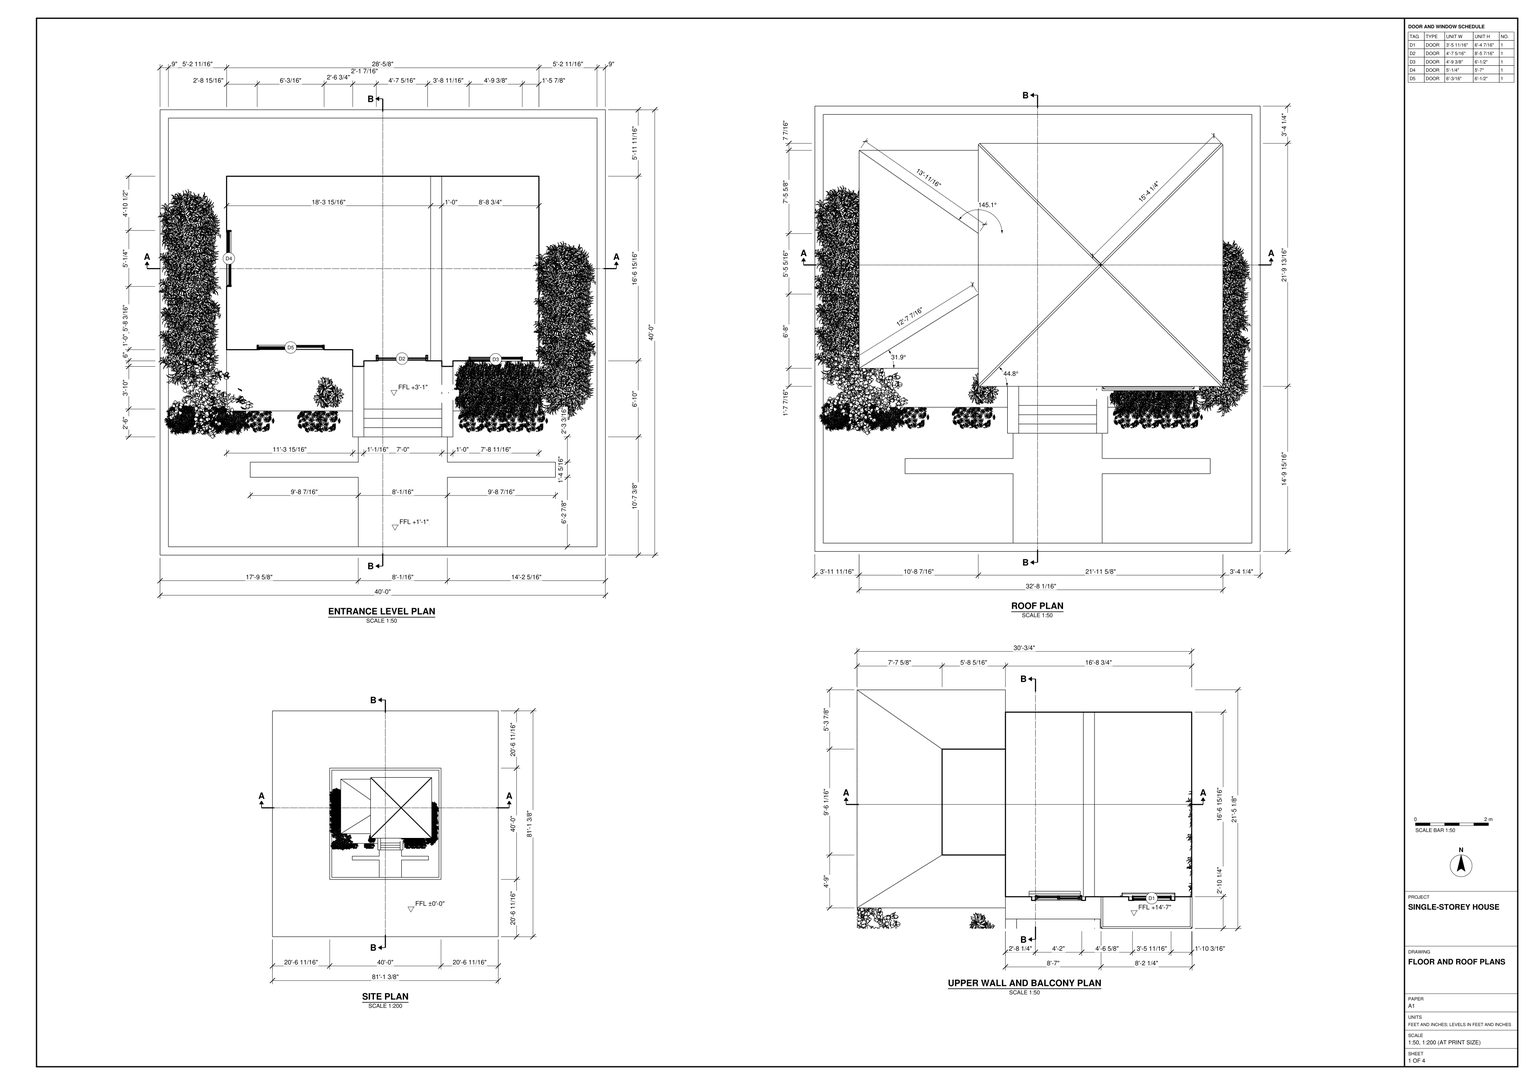
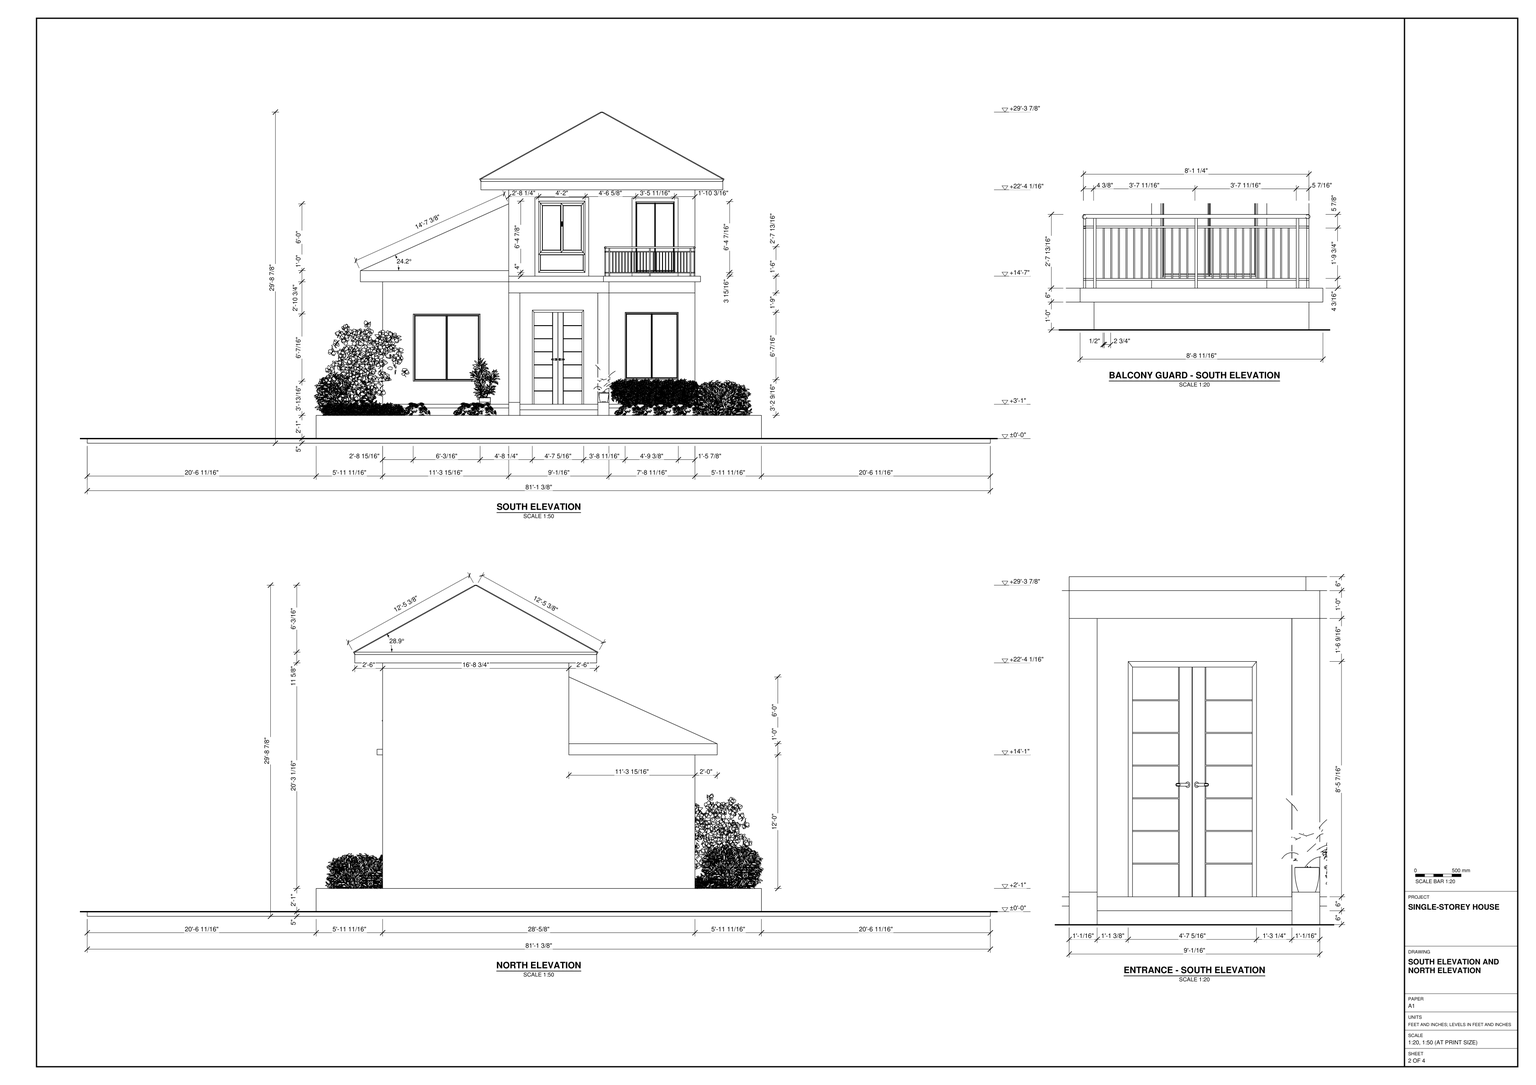
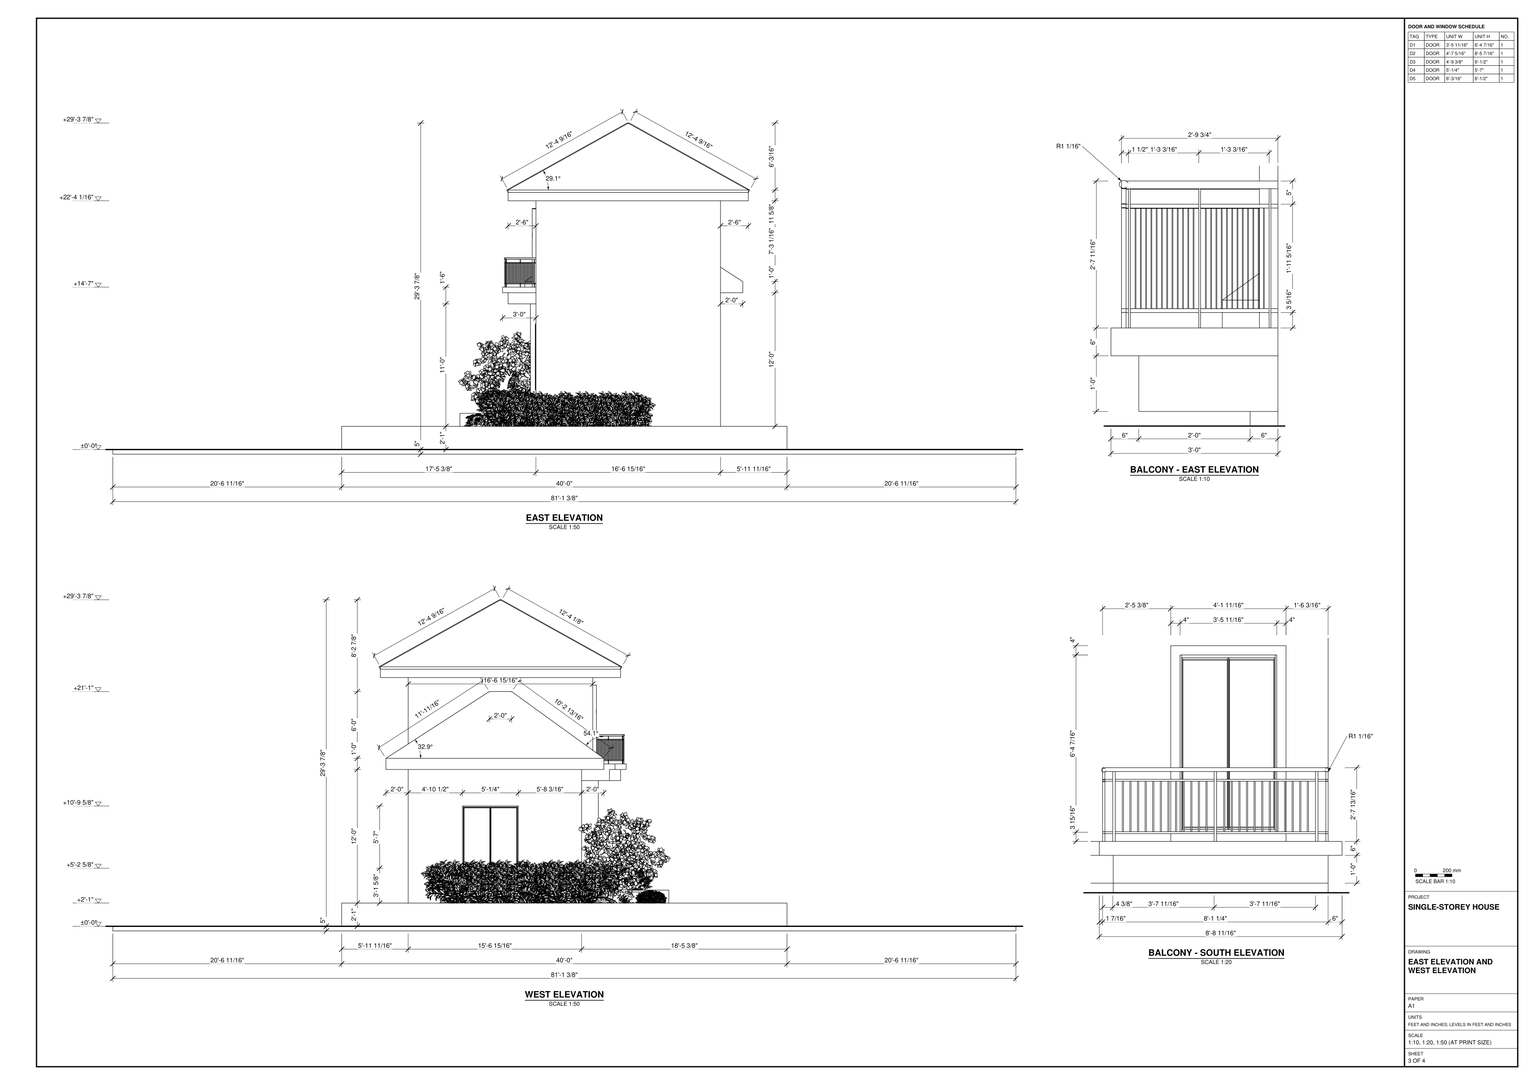
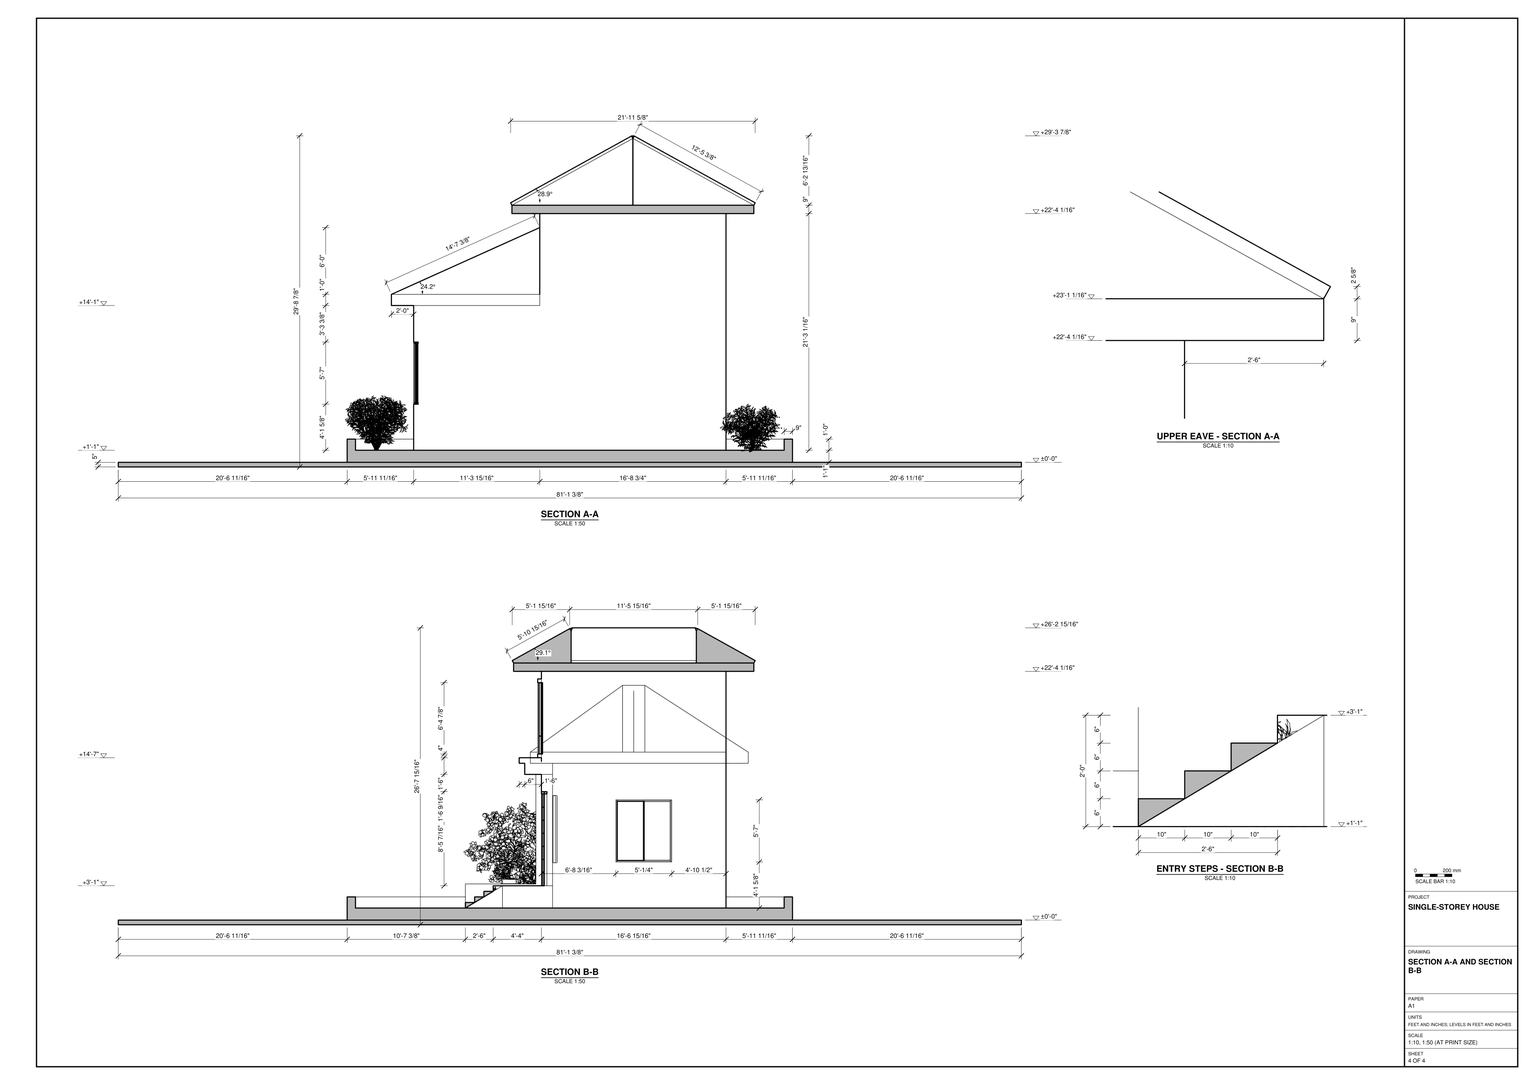
Build the house and its site in SketchUp from task_files/diagram_01.pdf. Work in feet and inches. Use the site datum of ±0'-0". The complete model, including the base slab, must measure 81'-1 3/8" along both plan axes and 29'-8 7/8" from the underside of the base to the roof peak.

Centre the raised square plot on the larger site slab. Run the entrance path from the south edge of the plot to the steps and landing at the double entrance door. Follow the entrance plan for the wall positions and thicknesses, the offsets in the south facade and the widths of the openings. Fit the glazed units on either side of the entrance and in the west wall. Model the upper south window and the door onto the projecting balcony, including its slab, front guard and side returns.

Form the taller east roof with hips meeting at a single peak. Fit the lower west roof against the taller wall, matching the roof plan and the eave profiles in elevation. Place the planting in the beds shown around the house. Plants, decor and loose items may be suitable library components. Keep walls, slabs, roofs and individual joinery or furniture pieces in separate groups or components, and use components for repeated parts. Save one SketchUp model as output_files/single_storey_house_with_hipped_roofs_and_a_balcony.skp.

# SketchUp Ruby script. Lengths in inches.
U = 1.inch
M = Sketchup.active_model
def pt(a) = Geom::Point3d.new(a.map { |v| v * U })
def face(e, loops, mat)
  f = e.add_face(loops[0].map { |a| pt(a) })
  loops[1..].each { |l| e.add_face(l.map { |a| pt(a) }).erase! }
  f.material = f.back_material = mat if mat
  f
end
# faces: each face lists its corners as indices into pts; further lists are holes
def faces(e, pts, list, mat = nil) = list.each { |f| face(e, (f[0].is_a?(Array) ? f : [f]).map { |l| l.map { |i| pts[i] } }, mat) }
# xy, xz, yz: faces in a plane at the given z, y or x. An outline is a flat list of corners, or four numbers for a rectangle; further outlines are holes
def ring(l) = l.size == 4 ? [[l[0], l[1]], [l[2], l[1]], [l[2], l[3]], [l[0], l[3]]] : l.each_slice(2).to_a
def flat(e, list, mat, &to3) = list.each { |f| face(e, (f[0].is_a?(Array) ? f : [f]).map { |l| ring(l).map { |u, v| to3.(u, v) } }, mat) }
def xy(e, z, list, mat = nil) = flat(e, list, mat) { |x, y| [x, y, z] }
def xz(e, y, list, mat = nil) = flat(e, list, mat) { |x, z| [x, y, z] }
def yz(e, x, list, mat = nil) = flat(e, list, mat) { |y, z| [x, y, z] }
def lines(e, pts, list) = list.each { |a, b| e.add_line(pt(pts[a]), pt(pts[b])) }
# prism: a flat outline (further loops are holes) pulled along v
def prism(e, loops, v, mat = nil)
  f = face(e, loops, mat); d = Geom::Vector3d.new(v.map { |x| x * U })
  f.pushpull(f.normal.samedirection?(d) ? d.length : -d.length)
end
def box(e, o, s, mat = nil) = prism(e, [[o, [o[0] + s[0], o[1], o[2]], [o[0] + s[0], o[1] + s[1], o[2]], [o[0], o[1] + s[1], o[2]]]], [0, 0, s[2]], mat)
def at(x, y, z, deg = 0) = Geom::Transformation.translation(pt([x, y, z])) * Geom::Transformation.rotation(ORIGIN, Z_AXIS, deg.degrees)
def axes(o, x, y, z) = Geom::Transformation.new([*x, 0, *y, 0, *z, 0, *pt(o).to_a, 1])
def part(name) = M.definitions.add(name)
# library, detail: a bought-in or finely detailed component or shape, given as its bounding box
def library(name, o, s) = part(name).tap { |d| box(d.entities, o, s) }
def detail(e, o, s) = box(e.add_group.entities, o, s)
def put(e, d, t, mat = nil) = e.add_instance(d, t).tap { |i| i.material = mat if mat }
def group(e, t, mat = nil) = e.add_group.tap { |g| g.transformation = t; g.material = mat if mat }.entities
root = M.entities
M.materials.add("Glass_Tinted_Gray").color = [0, 0, 0]
M.materials["Glass_Tinted_Gray"].alpha = 0.125
M.materials.add("[0045_Goldenrod]").color = [218, 165, 32]
M.materials.add("[0053_Ivory]").color = [255, 255, 240]
M.materials.add("[0135_DarkGray]").color = [81, 81, 81]
M.materials.add("[Color M06]1").color = [86, 86, 86]
M.materials.add("[Color_F16]").color = [51, 102, 0]
M.materials.add("[Granite Light Gray]1").color = [114, 113, 110]
M.materials.add("[Granite Light Gray]2").color = [112, 111, 107]
M.materials.add("[Grass Dark Green]").color = [98, 145, 50]
M.materials.add("[Mirror 02]").color = [229, 229, 229]
M.materials.add("[Pavers with Grass Brick]").color = [216, 221, 203]
M.materials.add("[Roofing Metal Standing Seam Red]1").color = [166, 70, 58]
M.materials.add("[Terrazzo Light Blue]").color = [196, 214, 227]
M.materials.add("[Wood Veneer 01]").color = [171, 112, 73]
c1 = library("Window with transom",[0,0,0],[5.2,55.12,70.87])
c2 = part("PENTEK_RP Fineline 50S_Sliding_DoorCase_E1")
box(c2.entities,[0,0,0],[1.51,3.66,99.27],"[0135_DarkGray]")
c3 = part("PENTEK_RP Fineline 50S_SlidingDooe_Case_E2")
box(c3.entities,[0,0,0],[96.25,3.66,1.51],"[0135_DarkGray]")
c4 = part("pentek_RP Fineline 50S_SlidingDoor_Case")
put(c4.entities,c2,at(97.76,0,0))
put(c4.entities,c3,at(1.51,0,0))
put(c4.entities,c2,at(0,0,0))
put(c4.entities,c3,at(1.51,0,97.76))
c5 = part("PENTEK_RP Fineline 50S_SlidingDoor_GlazingBead_2")
box(c5.entities,[0,0,0],[0.56,0.59,94.39],"[0135_DarkGray]")
c6 = part("PENTEK_RP Fineline 50S_SlidingDoor_Glass")
box(c6.entities,[0,0,0],[46.58,0.16,94.39],"Glass_Tinted_Gray")
c7 = part("PENTEK_RP Fineline 50S_SlidingDoor_GlazingBead")
box(c7.entities,[0,0,0],[45.47,0.59,0.56],"[0135_DarkGray]")
c8 = part("PENTEK_RP Fineline 50S_SlidingDoor_Leaf_E1")
xy(c8.entities,0,[[0,0,0.93,1.97],[0.93,1.57,1.49,1.97]],"[0135_DarkGray]")
xy(c8.entities,96.25,[[0,0,0.93,0,0.93,1.57,1.49,1.57,1.49,1.97,0,1.97]],"[0135_DarkGray]")
xz(c8.entities,0,[[0,0,0.93,96.25]],"[0135_DarkGray]")
xz(c8.entities,1.57,[[0.93,0,1.49,95.32],[0.93,95.32,1.49,96.25]],"[0135_DarkGray]")
xz(c8.entities,1.97,[[0,0,1.49,96.25]],"[0135_DarkGray]")
yz(c8.entities,0,[[0,0,1.97,96.25]],"[0135_DarkGray]")
yz(c8.entities,0.93,[[0,0,1.57,0.93],[0,0.93,1.57,95.32],[0,95.32,1.57,96.25]],"[0135_DarkGray]")
yz(c8.entities,1.49,[[1.57,0,1.97,95.32],[1.57,95.32,1.97,96.25]],"[0135_DarkGray]")
c9 = part("PENTEK_RP Fineline 50S_SlidingDoor_Leaf_E2")
xy(c9.entities,0,[[0,0,0,1.57,0.56,1.57,0.56,1.97,46.02,1.97,46.02,1.57,46.58,1.57,46.58,0]],"[0135_DarkGray]")
xy(c9.entities,0.93,[[0,0,46.58,1.57]],"[0135_DarkGray]")
xy(c9.entities,1.49,[[0.56,1.57,46.02,1.97]],"[0135_DarkGray]")
xz(c9.entities,0,[[0,0,46.58,0.93]],"[0135_DarkGray]")
xz(c9.entities,1.57,[[0,0,0.56,0.93],[46.02,0,46.58,0.93],[0.56,0.93,46.02,1.49]],"[0135_DarkGray]")
xz(c9.entities,1.97,[[0.56,0,46.02,1.49]],"[0135_DarkGray]")
yz(c9.entities,0,[[0,0,1.57,0.93]],"[0135_DarkGray]")
yz(c9.entities,0.56,[[1.57,0,1.97,0.93],[1.57,0.93,1.97,1.49]],"[0135_DarkGray]")
yz(c9.entities,46.02,[[1.57,0,1.97,0.93],[1.57,0.93,1.97,1.49]],"[0135_DarkGray]")
yz(c9.entities,46.58,[[0,0,1.57,0.93]],"[0135_DarkGray]")
c10 = part("PENTEK_RP Fineline S_SlidingDoor_Leaf1")
put(c10.entities,c5,at(0.93,0,0.93))
put(c10.entities,c5,at(46.96,0,0.93))
put(c10.entities,c6,at(1.49,1.42,0.93))
put(c10.entities,c7,at(1.49,0,0.93))
put(c10.entities,c6,at(1.49,0.59,0.93),"[Terrazzo Light Blue]")
put(c10.entities,c8,at(0,0,0))
put(c10.entities,c8,axes([48.44,0,0],[-1,0,0],[0,1,0],[0,0,1]))
put(c10.entities,c9,axes([0.93,0,96.25],[1,0,0],[0,1,0],[0,0,-1]))
put(c10.entities,c9,at(0.93,0,0))
put(c10.entities,c7,at(1.49,0,94.77))
c11 = part("PENTEK_RP Fineline 50S_SlidingDoor_Leaf2")
put(c11.entities,c6,at(1.49,1.42,0.93))
put(c11.entities,c7,at(1.49,0,94.77))
put(c11.entities,c5,at(46.96,0,0.93))
put(c11.entities,c6,at(1.49,0.59,0.93),"[Mirror 02]")
put(c11.entities,c5,at(0.93,0,0.93))
put(c11.entities,c8,at(0,0,0))
put(c11.entities,c8,axes([48.44,0,0],[-1,0,0],[0,1,0],[0,0,1]))
put(c11.entities,c7,at(1.49,0,0.93))
put(c11.entities,c9,axes([0.93,0,96.25],[1,0,0],[0,1,0],[0,0,-1]))
put(c11.entities,c9,at(0.93,0,0))
c12 = part("PENTEK - Slimmest Steel Sliding Door / Window\#1")
put(c12.entities,c4,at(0,-1.88,-0.09))
put(c12.entities,c10,at(1.51,-2.27,1.42))
put(c12.entities,c11,at(49.32,-0.3,1.42))
c13 = library("DOUBLE+DOOR",[0,-1.0625,0],[59.06,6.97,82.68])
c14 = part("Balcony handrail")
prism(c14.entities,[[[-4.92,1.68,0.29],[-4.92,1.48,0.13],[-4.92,1.24,0.03],[-4.92,0.98,0],[-4.92,0.73,0.03],[-4.92,0.49,0.13],[-4.92,0.29,0.29],[-4.92,0.13,0.49],[-4.92,0.03,0.73],[-4.92,0,0.98],[-4.92,0.03,1.24],[-4.92,0.13,1.48],[-4.92,0.29,1.68],[-4.92,0.49,1.84],[-4.92,0.73,1.93],[-4.92,0.98,1.97],[-4.92,1.24,1.93],[-4.92,1.48,1.84],[-4.92,1.68,1.68],[-4.92,1.84,1.48],[-4.92,1.93,1.24],[-4.92,1.97,0.98],[-4.92,1.93,0.73],[-4.92,1.84,0.49]]],[87.6,0,0],"[Color M06]1")
c15 = part("Railing post")
box(c15.entities,[0,0,0],[0.98,0.98,35.43],"[Color M06]1")
c16 = part("Railing baluster")
prism(c16.entities,[[[0,0.24,0],[0.01,0.3,0],[0.03,0.35,0],[0.07,0.4,0],[0.12,0.44,0],[0.18,0.46,0],[0.24,0.47,0],[0.3,0.46,0],[0.35,0.44,0],[0.4,0.4,0],[0.44,0.35,0],[0.46,0.3,0],[0.47,0.24,0],[0.46,0.18,0],[0.44,0.12,0],[0.4,0.07,0],[0.35,0.03,0],[0.3,0.01,0],[0.24,0,0],[0.18,0.01,0],[0.12,0.03,0],[0.07,0.07,0],[0.03,0.12,0],[0.01,0.18,0]]],[0,0,25.59],"[Color M06]1")
c17 = part("Horizontal railing bar")
box(c17.entities,[0,0,0],[38.39,0.98,0.98],"[Color M06]1")
c18 = part("Component\#1")
box(c18.entities,[0,0,0],[0.98,0.98,3.9375],"[Color M06]1")
c19 = part("vertical+railing")
g1 = group(c19.entities,at(0,0,0))
p = [[4.92,0.49,0],[4.92,0.49,3.9375]]
lines(g1,p,[[0,1]])
put(g1,c14,at(4.92,0,35.43))
g2 = group(g1,at(3.9375,0.49,0))
put(g2,c15,axes([40.35,0,0],[-1,0,0],[0,1,0],[0,0,1]))
put(g2,c15,axes([79.72,0,0],[-1,0,0],[0,1,0],[0,0,1]))
put(g2,c15,at(0,0,0))
g3 = group(g1,at(79.96,0.75,4.92))
put(g3,c16,axes([-29.53,0,0],[-1,0,0],[0,1,0],[0,0,1]))
put(g3,c16,axes([-23.62,0,0],[-1,0,0],[0,1,0],[0,0,1]))
put(g3,c16,axes([-17.72,0,0],[-1,0,0],[0,1,0],[0,0,1]))
put(g3,c16,axes([-20.67,0,0],[-1,0,0],[0,1,0],[0,0,1]))
put(g3,c16,axes([-26.57,0,0],[-1,0,0],[0,1,0],[0,0,1]))
put(g3,c16,axes([-11.8125,0,0],[-1,0,0],[0,1,0],[0,0,1]))
put(g3,c16,axes([-2.95,0,0],[-1,0,0],[0,1,0],[0,0,1]))
put(g3,c16,axes([-8.86,0,0],[-1,0,0],[0,1,0],[0,0,1]))
put(g3,c16,axes([-14.76,0,0],[-1,0,0],[0,1,0],[0,0,1]))
put(g3,c16,axes([-32.48,0,0],[-1,0,0],[0,1,0],[0,0,1]))
put(g3,c16,axes([0,0,0],[-1,0,0],[0,1,0],[0,0,1]))
put(g3,c16,axes([-5.91,0,0],[-1,0,0],[0,1,0],[0,0,1]))
g4 = group(g1,at(82.68,0.49,3.9375))
put(g4,c17,axes([0,0,0],[-1,0,0],[0,1,0],[0,0,1]))
put(g4,c17,axes([0,0,26.57],[-1,0,0],[0,1,0],[0,0,1]))
g5 = group(g1,at(0,0.49,3.9375))
put(g5,c18,axes([83.66,0,0],[0,0,1],[0,1,0],[1,0,0]))
put(g5,c18,axes([83.66,0,26.57],[0,0,1],[0,1,0],[1,0,0]))
put(g5,c18,axes([3.9375,0,26.57],[0,0,1],[0,1,0],[-1,0,0]))
put(g5,c18,axes([3.9375,0,0],[0,0,1],[0,1,0],[-1,0,0]))
g6 = group(g1,at(4.92,0.49,3.9375))
put(g6,c17,at(0,0,0))
put(g6,c17,at(0,0,26.57))
g7 = group(g1,at(7.64,0.75,4.92))
put(g7,c16,at(29.53,0,0))
put(g7,c16,at(23.62,0,0))
put(g7,c16,at(17.72,0,0))
put(g7,c16,at(20.67,0,0))
put(g7,c16,at(26.57,0,0))
put(g7,c16,at(11.8125,0,0))
put(g7,c16,at(2.95,0,0))
put(g7,c16,at(8.86,0,0))
put(g7,c16,at(14.76,0,0))
put(g7,c16,at(32.48,0,0))
put(g7,c16,at(0,0,0))
put(g7,c16,at(5.91,0,0))
c20 = library("Obj_000003",[-31,-31.06,-7.89],[62,62.12,39.58])
c21 = library("Obj_000004",[-25.54,-25.36,-14.31],[50.67,50.64,41.42])
c22 = part("Sin+título")
put(c22.entities,c20,at(175.17,79.15,26.91,103.6),"[Color_F16]")
put(c22.entities,c20,axes([175.17,78.65,14.31],[-0.2647,0.96433,-0.00055],[-0.96433,-0.2647,0.00023],[0.00007,0.00059,1]),"[Color_F16]")
put(c22.entities,c20,axes([175.13,79.8,26.91],[-0.85355,0.52101,-0.00055],[-0.52101,-0.85355,0.00023],[-0.00035,0.00048,1]),"[Color_F16]")
put(c22.entities,c21,at(175.17,79.15,26.91,103.6))
put(c22.entities,c21,axes([175.17,78.65,14.31],[-0.2647,0.96433,-0.00055],[-0.96433,-0.2647,0.00023],[0.00007,0.00059,1]))
put(c22.entities,c21,axes([200.01,78.32,26.91],[0.70711,0.70711,-0.00055],[-0.70711,0.70711,0.00023],[0.00055,0.00023,1]))
put(c22.entities,c21,at(124.96,78.44,26.91))
put(c22.entities,c21,at(149.76,78.44,14.31))
put(c22.entities,c20,axes([125.6,78.32,26.91],[0.70711,0.70711,-0.00055],[-0.70711,0.70711,0.00023],[0.00055,0.00023,1]),"[Color_F16]")
put(c22.entities,c20,axes([150.4,78.32,14.31],[0.70711,0.70711,-0.00055],[-0.70711,0.70711,0.00023],[0.00055,0.00023,1]),"[Color_F16]")
put(c22.entities,c20,at(124.96,78.44,14.31),"[Color_F16]")
put(c22.entities,c20,at(124.96,78.44,26.91),"[Color_F16]")
put(c22.entities,c21,axes([125.6,78.32,14.31],[0.70711,0.70711,-0.00055],[-0.70711,0.70711,0.00023],[0.00055,0.00023,1]))
put(c22.entities,c21,at(124.96,78.44,14.31))
put(c22.entities,c20,axes([247.77,77.22,14.31],[0.53367,0.84569,-0.00055],[-0.84569,0.53367,0.00023],[0.00049,0.00034,1]),"[Color_F16]")
put(c22.entities,c21,axes([248.92,79.375,26.91],[-0.32227,0.94665,-0.00055],[-0.94665,-0.32227,0.00023],[0.00004,0.0006,1]))
put(c22.entities,c20,at(248.53,78.85,14.31,63.8),"[Color_F16]")
put(c22.entities,c20,axes([224.8125,78.32,14.31],[0.70711,0.70711,-0.00055],[-0.70711,0.70711,0.00023],[0.00055,0.00023,1]),"[Color_F16]")
put(c22.entities,c21,at(224.17,78.44,14.31))
put(c22.entities,c20,at(224.17,78.44,26.91),"[Color_F16]")
put(c22.entities,c21,at(248.53,78.85,26.91,63.8))
put(c22.entities,c21,axes([247.77,77.22,14.31],[0.53367,0.84569,-0.00055],[-0.84569,0.53367,0.00023],[0.00049,0.00034,1]))
put(c22.entities,c21,at(248.53,78.85,14.31,63.8))
put(c22.entities,c20,at(248.98,78.44,26.91),"[Color_F16]")
put(c22.entities,c20,axes([248.92,79.375,26.91],[-0.32227,0.94665,-0.00055],[-0.94665,-0.32227,0.00023],[0.00004,0.0006,1]),"[Color_F16]")
put(c22.entities,c21,axes([150.4,78.32,26.91],[0.70711,0.70711,-0.00055],[-0.70711,0.70711,0.00023],[0.00055,0.00023,1]))
put(c22.entities,c21,at(199.37,78.44,26.91))
put(c22.entities,c21,axes([150.4,78.32,14.31],[0.70711,0.70711,-0.00055],[-0.70711,0.70711,0.00023],[0.00055,0.00023,1]))
put(c22.entities,c20,axes([200.01,78.32,14.31],[0.70711,0.70711,-0.00055],[-0.70711,0.70711,0.00023],[0.00055,0.00023,1]),"[Color_F16]")
put(c22.entities,c21,axes([200.01,78.32,14.31],[0.70711,0.70711,-0.00055],[-0.70711,0.70711,0.00023],[0.00055,0.00023,1]))
put(c22.entities,c21,at(199.37,78.44,14.31))
put(c22.entities,c20,axes([200.01,78.32,26.91],[0.70711,0.70711,-0.00055],[-0.70711,0.70711,0.00023],[0.00055,0.00023,1]),"[Color_F16]")
put(c22.entities,c20,at(175.17,79.15,14.31,103.6),"[Color_F16]")
put(c22.entities,c21,at(175.17,79.15,14.31,103.6))
put(c22.entities,c21,axes([175.13,79.8,26.91],[-0.85355,0.52101,-0.00055],[-0.52101,-0.85355,0.00023],[-0.00035,0.00048,1]))
put(c22.entities,c21,axes([125.6,78.32,26.91],[0.70711,0.70711,-0.00055],[-0.70711,0.70711,0.00023],[0.00055,0.00023,1]))
put(c22.entities,c20,axes([150.4,78.32,26.91],[0.70711,0.70711,-0.00055],[-0.70711,0.70711,0.00023],[0.00055,0.00023,1]),"[Color_F16]")
put(c22.entities,c21,at(149.76,78.44,26.91))
put(c22.entities,c20,at(149.76,78.44,26.91),"[Color_F16]")
put(c22.entities,c20,at(149.76,78.44,14.31),"[Color_F16]")
put(c22.entities,c20,at(199.37,78.44,14.31),"[Color_F16]")
put(c22.entities,c20,at(199.37,78.44,26.91),"[Color_F16]")
put(c22.entities,c21,axes([224.8125,78.32,14.31],[0.70711,0.70711,-0.00055],[-0.70711,0.70711,0.00023],[0.00055,0.00023,1]))
put(c22.entities,c21,at(224.17,78.44,26.91))
put(c22.entities,c20,at(224.17,78.44,14.31),"[Color_F16]")
put(c22.entities,c21,axes([224.8125,78.32,26.91],[0.70711,0.70711,-0.00055],[-0.70711,0.70711,0.00023],[0.00055,0.00023,1]))
put(c22.entities,c20,axes([224.8125,78.32,26.91],[0.70711,0.70711,-0.00055],[-0.70711,0.70711,0.00023],[0.00055,0.00023,1]),"[Color_F16]")
c23 = library("Plant+(3) (1)",[-15.5,2.64,0],[117.71,96.38,184.75])
c24 = library("Plant Decor 06",[-19.54,-17.78,0],[35.83,37.65,42.54])
c25 = library("tree07",[-42.875,-48.82,0],[95.28,102.01,116.69])
c26 = library("Knockout Roses",[-32.26,14.89,-3.45],[37.25,36.64,34.74])
xy(root,0,[[0,0,973.375,973.375]])
xy(root,5.01,[[246.6875,246.6875,726.6875,726.6875]])
xy(root,5.01,[[[0,0,973.375,973.375],[246.6875,246.6875,726.6875,726.6875]]],"[Wood Veneer 01]")
xy(root,18,[[454.28,374.09,466.35,374.09,466.35,414.09,550.35,414.09,550.35,374.09,562.35,374.09,562.35,404.09,655.01,404.09,655.01,655.01,318.37,655.01,318.37,404.09,454.28,404.09],[466.35,374.09,550.35,414.09]])
xy(root,18,[[255.6875,255.6875,460.32,255.6875,460.32,330.57,343.88,330.57,343.88,346.88,460.32,346.88,460.32,374.09,454.28,374.09,454.28,404.09,318.37,404.09,318.37,655.01,655.01,655.01,655.01,404.09,562.35,404.09,562.35,374.09,556.35,374.09,556.35,346.88,672.79,346.88,672.79,330.57,556.35,330.57,556.35,255.6875,717.6875,255.6875,717.6875,717.6875,255.6875,717.6875]],"[Grass Dark Green]")
xy(root,18,[[460.32,255.6875,556.35,255.6875,556.35,330.57,672.79,330.57,672.79,346.88,556.35,346.88,556.35,374.09,460.32,374.09,460.32,346.88,343.88,346.88,343.88,330.57,460.32,330.57]],"[Pavers with Grass Brick]")
xy(root,24,[[466.35,374.09,550.35,384.09]],"[Granite Light Gray]1")
xy(root,30,[[[246.6875,246.6875,726.6875,726.6875],[255.6875,255.6875,717.6875,717.6875]]],"[0053_Ivory]")
xy(root,30,[[466.35,384.09,550.35,394.09]],"[Granite Light Gray]1")
xy(root,36,[[466.35,394.09,550.35,404.09],[572.375,413.8,646.9375,444.82]],"[Granite Light Gray]1")
xy(root,38,[[318.37,402.09,454.28,404.09],[562.35,402.09,655.01,404.09]],"[Granite Light Gray]1")
xy(root,42,[[318.37,402.09,454.28,468.09],[[562.35,402.09,655.01,456.09],[572.375,413.8,646.9375,444.82]],[466.35,404.09,550.35,404.09,550.35,456.09,535.06,456.09,535.06,459.09,479.75,459.09,479.75,456.09,466.35,456.09]],"[Granite Light Gray]1")
xy(root,44,[[454.28,374.09,466.35,450.09],[550.35,374.09,562.35,450.09]],"[Granite Light Gray]1")
xy(root,66.86,[[351.33,468.09,423.52,471.09]])
xy(root,67.625,[[318.37,536.28,321.37,596.53]])
xy(root,68.55,[[579.72,456.09,637.125,459.09]])
xy(root,134.625,[[318.37,536.28,321.37,596.53]])
xy(root,139.05,[[351.33,468.09,423.52,471.09]])
xy(root,140.74,[[579.72,456.09,637.125,459.09]])
xy(root,143.4375,[[479.75,456.09,535.06,459.09]])
xy(root,162,[[562.35,426.09,562.35,438.09,454.28,438.09,454.28,450.09,466.35,450.09,466.35,456.09,550.35,456.09,550.35,450.09,562.35,450.09,562.35,456.09,655.01,456.09,655.01,426.09]],"[0053_Ivory]")
xy(root,174,[[556.35,420.09,556.35,432.09,454.28,432.09,454.28,438.09,562.35,438.09,562.35,426.09,655.01,426.09,655.01,456.09,661.01,456.09,661.01,420.09],[294.37,444.09,294.37,679.01,454.28,679.01,454.28,655.01,318.37,655.01,318.37,468.09,454.28,468.09,454.28,444.09]],"[0053_Ivory]")
xy(root,180,[[482.53,452.09,486.53,456.09],[486.53,452.09,536.53,456.09],[536.53,452.09,540.53,456.09],[587.15,452.09,591.15,456.09],[591.15,452.09,632.84,456.09],
  [632.84,452.09,636.84,456.09]])
xy(root,180,[[556.35,420.09,661.01,420.09,661.01,456.09,636.84,456.09,636.84,452.09,587.15,452.09,587.15,456.09,540.53,456.09,540.53,452.09,482.53,452.09,482.53,456.09,454.28,456.09,454.28,432.09,556.35,432.09]],"[0053_Ivory]")
xy(root,184,[[486.53,452.09,536.53,456.09],[591.15,452.09,632.84,456.09]],"[0053_Ivory]")
xy(root,260.375,[[591.15,452.09,632.84,456.09]])
xy(root,260.9,[[486.53,452.09,536.53,456.09]])
xy(root,264.375,[[587.15,452.09,636.84,456.09]],"[0053_Ivory]")
xy(root,264.9,[[482.53,452.09,540.53,456.09]],"[0053_Ivory]")
xy(root,273.0625,[[454.28,456.09,655.01,655.01]])
xy(root,273.0625,[[[424.28,426.09,685.01,685.01],[454.28,456.09,655.01,655.01]]],"[0053_Ivory]")
xy(root,282.0625,[[424.28,426.09,554.65,555.55,424.28,685.01],[424.28,426.09,685.01,426.09,554.65,555.55],[685.01,426.09,685.01,685.01,554.65,555.55],[554.65,555.55,685.01,685.01,424.28,685.01]])
xz(root,0,[[0,0,973.375,5.01]])
xz(root,246.6875,[[246.6875,5.01,726.6875,30]],"[0053_Ivory]")
xz(root,255.6875,[[255.6875,18,460.32,30],[460.32,18,556.35,30],[556.35,18,717.6875,30]],"[0053_Ivory]")
xz(root,374.09,[[454.28,18,466.35,44],[466.35,18,550.35,24],[550.35,18,562.35,44]],"[Granite Light Gray]1")
xz(root,384.09,[[466.35,24,550.35,30]],"[Granite Light Gray]1")
xz(root,394.09,[[466.35,30,550.35,36]],"[Granite Light Gray]1")
xz(root,402.09,[[318.37,38,454.28,42],[562.35,38,655.01,42]],"[Granite Light Gray]1")
xz(root,404.09,[[318.37,18,454.28,38],[562.35,18,655.01,38],[466.35,36,550.35,42]],"[Granite Light Gray]1")
xz(root,413.8,[[572.375,36,646.9375,42]],"[Granite Light Gray]1")
xz(root,420.09,[[556.35,174,661.01,180]],"[0053_Ivory]")
xz(root,426.09,[[562.35,162,655.01,174],[424.28,273.0625,685.01,282.0625]],"[0053_Ivory]")
xz(root,432.09,[[454.28,174,556.35,180]],"[0053_Ivory]")
xz(root,438.09,[[454.28,162,562.35,174]],"[0053_Ivory]")
xz(root,444.09,[[294.37,174,454.28,186]],"[0053_Ivory]")
xz(root,444.82,[[572.375,36,646.9375,42]],"[Granite Light Gray]1")
xz(root,450.09,[[454.28,44,466.35,162],[550.35,44,562.35,162]],"[Granite Light Gray]1")
xz(root,452.09,[[[482.53,180,540.53,264.9],[486.53,184,536.53,260.9]],[[587.15,180,636.84,264.375],[591.15,184,632.84,260.375]]],"[0053_Ivory]")
xz(root,456.09,[[550.28,42,550.35,162],[482.53,176,540.53,180],[587.15,176,636.84,180]])
xz(root,456.09,[[486.53,184,536.53,260.9],[591.15,184,632.84,260.375]],"[0045_Goldenrod]")
xz(root,456.09,[[466.35,42,479.75,42,479.75,143.4375,535.06,143.4375,535.06,42,550.28,42,550.28,162,466.35,162],[[562.35,42,655.01,162],[579.72,68.55,637.125,140.74]],[655.01,174,661.01,180],[454.28,180,482.53,180,482.53,264.9,540.53,264.9,540.53,180,587.15,180,587.15,264.375,636.84,264.375,636.84,180,655.01,180,655.01,273.0625,454.28,273.0625]],"[0053_Ivory]")
xz(root,459.09,[[479.75,42,535.06,143.4375]])
xz(root,459.09,[[579.72,68.55,637.125,140.74]],"[0045_Goldenrod]")
xz(root,468.09,[[[318.37,42,454.28,174],[351.33,66.86,423.52,139.05]]],"[0053_Ivory]")
xz(root,471.09,[[351.33,66.86,423.52,139.05]],"[0045_Goldenrod]")
xz(root,536.28,[[318.37,67.625,321.37,134.625]])
xz(root,596.53,[[318.37,67.625,321.37,134.625]])
xz(root,655.01,[[318.37,18,318.37,174,454.28,174,454.28,273.0625,655.01,273.0625,655.01,18]],"[0053_Ivory]")
xz(root,679.01,[[294.37,174,454.28,186]])
xz(root,685.01,[[424.28,273.0625,685.01,282.0625]],"[0053_Ivory]")
xz(root,717.6875,[[255.6875,18,717.6875,30]],"[0053_Ivory]")
xz(root,726.6875,[[246.6875,5.01,726.6875,30]],"[0053_Ivory]")
xz(root,973.375,[[0,0,973.375,5.01]])
yz(root,0,[[0,0,973.375,5.01]])
yz(root,246.6875,[[246.6875,5.01,726.6875,30]],"[0053_Ivory]")
yz(root,255.6875,[[255.6875,18,717.6875,30]],"[0053_Ivory]")
yz(root,294.37,[[444.09,174,679.01,186]],"[0053_Ivory]")
yz(root,318.37,[[[468.09,18,655.01,174],[536.28,67.625,596.53,134.625]]],"[0053_Ivory]")
yz(root,318.37,[[404.09,18,404.09,38,402.09,38,402.09,42,468.09,42,468.09,18]],"[Granite Light Gray]2")
yz(root,321.37,[[536.28,67.625,596.53,134.625]],"[0045_Goldenrod]")
yz(root,351.33,[[468.09,66.86,471.09,139.05]])
yz(root,423.52,[[468.09,66.86,471.09,139.05]])
yz(root,424.28,[[426.09,273.0625,685.01,282.0625]],"[0053_Ivory]")
yz(root,454.28,[[655.01,174,679.01,174,679.01,186,655.01,201.5],[456.09,186,456.09,194.6875,543.55,258,543.55,186],[543.55,186,567.55,258],[567.55,186,567.55,258,655.01,201.5,655.01,186]])
yz(root,454.28,[[438.09,162,438.09,174,432.09,174,432.09,180,444.09,180,444.09,174,468.09,174,468.09,162],[444.09,180,456.09,186],[444.09,186,456.09,186,456.09,194.6875],[456.09,194.6875,456.09,273.0625,655.01,273.0625,655.01,201.5,567.55,258,543.55,258]],"[0053_Ivory]")
yz(root,454.28,[[374.09,18,374.09,44,450.09,44,450.09,162,468.09,162,468.09,42,402.09,42,402.09,38,404.09,38,404.09,18]],"[Granite Light Gray]1")
yz(root,466.35,[[374.09,18,384.09,24,374.09,24],[374.09,18,414.09,18,414.09,42],[384.09,24,384.09,30,394.09,30],[384.09,24,402.09,34.8,394.09,34.8,394.09,30,384.09,30],[394.09,34.8,402.09,36]])
yz(root,466.35,[[374.09,24,384.09,24,384.09,30,394.09,30,394.09,36,404.09,36,404.09,42,456.09,42,456.09,162,450.09,162,450.09,44,374.09,44]],"[Granite Light Gray]1")
yz(root,479.75,[[456.09,42,459.09,143.4375]])
yz(root,482.53,[[452.09,180,456.09,264.9]],"[0053_Ivory]")
yz(root,486.53,[[452.09,184,456.09,260.9]],"[0053_Ivory]")
yz(root,535.06,[[456.09,42,459.09,143.4375]])
yz(root,536.53,[[452.09,184,456.09,260.9]],"[0053_Ivory]")
yz(root,540.53,[[452.09,180,456.09,264.9]],"[0053_Ivory]")
yz(root,550.35,[[374.09,18,374.09,24,384.09,24],[374.09,18,414.09,42,414.09,18],[384.09,24,384.09,30,394.09,30],[384.09,24,394.09,30,384.09,30],[394.09,30,394.09,34.8,402.09,34.8],
  [394.09,34.8,402.09,36],[402.09,34.8,404.09,36,402.09,36],[402.09,34.8,404.09,36,404.09,42,414.09,42,404.09,36,402.09,36],[404.09,36,404.09,42,414.09,42],[404.09,36,404.09,42,414.09,42]])
yz(root,550.35,[[374.09,24,374.09,44,450.09,44,450.09,162,456.09,162,456.09,42,404.09,42,404.09,36,394.09,36,394.09,30,384.09,30,384.09,24]],"[Granite Light Gray]1")
yz(root,556.35,[[420.09,174,432.09,180]],"[0053_Ivory]")
yz(root,562.35,[[426.09,162,438.09,174]],"[0053_Ivory]")
yz(root,562.35,[[374.09,18,404.09,18,404.09,38,402.09,38,402.09,42,456.09,42,456.09,162,450.09,162,450.09,44,374.09,44]],"[Granite Light Gray]1")
yz(root,572.375,[[413.8,36,444.82,42]],"[Granite Light Gray]1")
yz(root,579.72,[[456.09,68.55,459.09,140.74]])
yz(root,587.15,[[452.09,180,456.09,264.375]],"[0053_Ivory]")
yz(root,591.15,[[452.09,184,456.09,260.375]])
yz(root,632.84,[[452.09,184,456.09,260.375]])
yz(root,636.84,[[452.09,180,456.09,264.375]],"[0053_Ivory]")
yz(root,637.125,[[456.09,68.55,459.09,140.74]])
yz(root,646.9375,[[413.8,36,444.82,42]],"[Granite Light Gray]1")
yz(root,655.01,[[404.09,18,655.01,18,655.01,273.0625,456.09,273.0625,456.09,42,402.09,42,402.09,38,404.09,38],[426.09,162,456.09,174]],"[0053_Ivory]")
yz(root,661.01,[[420.09,174,456.09,180]],"[0053_Ivory]")
yz(root,685.01,[[426.09,273.0625,685.01,282.0625]],"[0053_Ivory]")
yz(root,717.6875,[[255.6875,18,717.6875,30]],"[0053_Ivory]")
yz(root,726.6875,[[246.6875,5.01,726.6875,30]],"[0053_Ivory]")
yz(root,973.375,[[0,0,973.375,5.01]])
p = [[466.35,374.09,18],[466.35,384.09,24],[550.35,384.09,24],[550.35,374.09,18],[466.35,394.09,30],[550.35,394.09,30],
  [466.35,402.09,34.8],[550.35,402.09,34.8],[466.35,404.09,36],[550.35,404.09,36],[454.28,543.55,258],[454.28,567.55,258],
  [294.37,679.01,186],[294.37,444.09,186],[454.28,456.09,194.6875],[454.28,444.09,186],[454.28,655.01,201.5],[454.28,679.01,186],
  [424.28,424.63,284.68],[422.83,426.09,284.6875],[424.28,426.09,282.0625],[554.65,555.55,354.0625],[554.65,554.09,356.68],[685.01,426.09,282.0625],
  [685.01,424.63,284.68],[686.46,426.09,284.6875],[424.28,685.01,282.0625],[422.83,685.01,284.6875],[553.2,555.55,356.6875],[554.65,555.55,282.0625],
  [556.1,555.55,356.6875],[685.01,685.01,282.0625],[686.46,685.01,284.6875],[554.65,557.01,356.68],[424.28,686.47,284.68],[685.01,686.47,284.68],
  [554.27,554.46,356.89],[554.27,555.55,354.93],[554.27,555.92,354.27],[555.02,555.92,354.27],[555.02,555.55,354.93],[555.02,554.46,356.89],
  [555.02,555.18,354.27],[554.65,555.18,354.94],[553.57,555.18,356.89],[554.27,555.18,354.27],[554.27,556.64,356.89],[555.72,555.18,356.89],
  [555.02,556.64,356.89],[553.57,555.92,356.89],[554.65,555.92,354.94],[555.72,555.92,356.89],[553.93,555.55,356.89],[554.65,554.83,356.89],
  [555.36,555.55,356.89],[554.65,556.26,356.89],[538.28,456.09,42],[538.28,655.01,42],[550.28,456.09,42],[550.28,655.01,42],
  [454.28,555.55,186],[454.28,555.55,240],[454.28,555.55,252]]
faces(root,p,[[0,1,2,3],[1,4,5,2],[4,6,7,5],[6,8,9,7],[21,20,18,22],[23,21,22,24],[20,21,28,19],[21,20,29],
  [23,21,29],[21,23,25,30],[21,26,27,28],[21,26,29],[26,21,33,34],[31,21,29],[21,31,35,33],[31,21,30,32],
  [35,32,31],[22,28,21],[21,22,36,37,38],[30,22,21],[28,21,42,43,44],[21,33,48,40,42],[28,33,21],[30,21,38,50,51],
  [33,30,21]])
faces(root,p,[[10,11,12,13],[14,10,13,15],[11,16,17,12],[18,19,20],[20,23,24,18],[25,24,23],[26,20,19,27],[23,31,32,25],
  [27,34,26],[31,26,34,35],[19,18,22,28],[24,22,18],[24,25,30,22],[28,27,19],[32,30,25],[34,27,28,33],
  [32,35,33,30],[34,33,35],[22,21,39,40,41],[33,21,45,37,46],[21,30,47,43,45],[21,28,49,50,39],[49,52,53,41,40,39,50],[54,51,50,38,37,36,53],
  [48,55,52,44,43,42,40],[47,54,55,46,37,45,43],[28,22,41,53,52,49],[22,30,51,54,53,36],[33,28,44,52,55,48],[30,33,46,55,54,47]],"[Roofing Metal Standing Seam Red]1")
lines(root,p,[[56,57],[58,59],[60,61],[61,62]])
put(root,c1,axes([536.53,457.28,260.9],[0,-1,0],[-0.90714,0,0],[0,0,-1.08517]))
put(root,c12,axes([579.72,458.02,68.62],[0.57821,0,0],[0,1.19,0],[0,0,0.73]))
put(root,c12,axes([351.33,470.79,66.86],[0.72717,0,0],[0,1.19,0],[0,0,0.73]))
put(root,c12,axes([591.15,454.79,184],[0.41993,0,0],[0,1.19,0],[0,0,0.77002]))
put(root,c12,axes([321.07,596.53,67.6875],[0,-0.60692,0],[1.19,0,0],[0,0,0.67491]))
put(root,c13,axes([479.75,456.09,42],[0.93663,0,0],[0,1,0],[0,0,1.22691]))
put(root,c19,axes([557.77,421.86,180],[1.11,0,0],[0,1,0],[0,0,0.85]))
put(root,c19,axes([655.5,422.36,180],[0,0.385,0],[-1,0,0],[0,0,0.847]))
put(root,c19,axes([559.25,422.36,180],[0,0.385,0],[-1,0,0],[0,0,0.84345]))
put(root,c22,at(760.96,303.67,9.21,90))
put(root,c23,axes([416.36,403.79,42],[0.27995,0,0],[0,0.355,0],[0,0,0.27]))
put(root,c24,at(556.35,421.53,44))
put(root,c25,at(295.95,420.04,18))
put(root,c22,axes([356.81,323.35,18.02],[0,1.12964,0],[-1,0,0],[0,0,1]))
put(root,c22,axes([708.64,503.4,35.9],[-0.51874,0,0],[0,-1,0],[0,0,0.5751]))
put(root,c22,axes([387.79,433.6,10.1875],[-0.48558,0,0],[0,-0.5146,0],[0,0,0.5751]))
put(root,c26,at(369.24,358.93,14.05))
put(root,c26,at(425.49,358.93,14.05))
put(root,c26,at(440.49,358.93,14.05))
put(root,c26,at(599.12,358.93,14.05))
put(root,c26,at(621.99,358.93,14.05))
put(root,c26,at(642.74,358.93,14.05))
put(root,c26,at(664.05,358.93,14.05))
